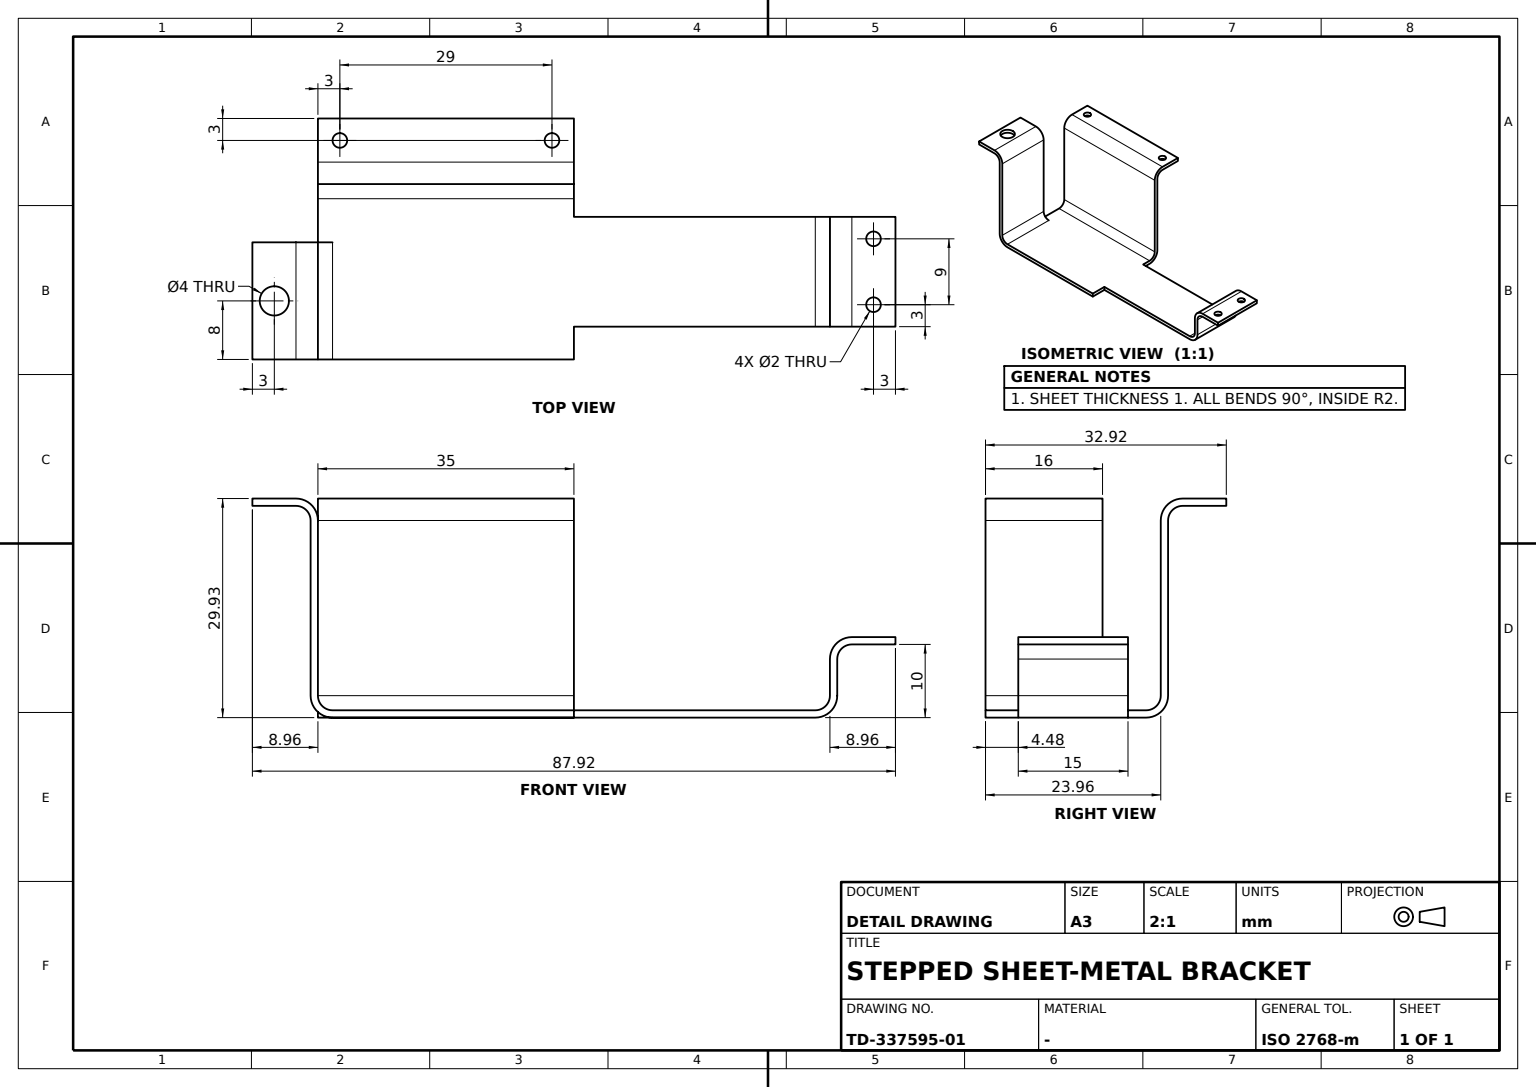
ISO-10303-21;
HEADER;
FILE_DESCRIPTION((''),'2;1');
FILE_NAME('','',(''),(''),'','','');
FILE_SCHEMA(('AUTOMOTIVE_DESIGN'));
ENDSEC;
DATA;
#1=APPLICATION_CONTEXT('');
#2=PRODUCT_CONTEXT('',#1,'mechanical');
#3=PRODUCT('','','',(#2));
#4=PRODUCT_DEFINITION_FORMATION('','',#3);
#5=PRODUCT_DEFINITION_CONTEXT('',#1,'design');
#6=PRODUCT_DEFINITION('','',#4,#5);
#7=PRODUCT_DEFINITION_SHAPE('','',#6);
#8=(LENGTH_UNIT()NAMED_UNIT(*)SI_UNIT(.MILLI.,.METRE.));
#9=(NAMED_UNIT(*)PLANE_ANGLE_UNIT()SI_UNIT($,.RADIAN.));
#10=(NAMED_UNIT(*)SI_UNIT($,.STERADIAN.)SOLID_ANGLE_UNIT());
#11=UNCERTAINTY_MEASURE_WITH_UNIT(LENGTH_MEASURE(0.005),#8,'distance_accuracy_value','');
#12=(GEOMETRIC_REPRESENTATION_CONTEXT(3)GLOBAL_UNCERTAINTY_ASSIGNED_CONTEXT((#11))GLOBAL_UNIT_ASSIGNED_CONTEXT((#8,#9,#10))REPRESENTATION_CONTEXT('',''));
#13=CARTESIAN_POINT('',(18.94,38.,29.93));
#14=VERTEX_POINT('',#13);
#15=CARTESIAN_POINT('',(17.94,38.,29.93));
#16=DIRECTION('',(0.,0.,1.));
#17=DIRECTION('',(1.,0.,0.));
#18=AXIS2_PLACEMENT_3D('',#15,#16,#17);
#19=CIRCLE('',#18,1.);
#20=EDGE_CURVE('',#14,#14,#19,.T.);
#21=ORIENTED_EDGE('',*,*,#20,.T.);
#22=EDGE_LOOP('',(#21));
#23=FACE_BOUND('',#22,.T.);
#24=CARTESIAN_POINT('',(18.94,38.,28.93));
#25=VERTEX_POINT('',#24);
#26=CARTESIAN_POINT('',(17.94,38.,28.93));
#27=AXIS2_PLACEMENT_3D('',#26,#16,#17);
#28=CIRCLE('',#27,1.);
#29=EDGE_CURVE('',#25,#25,#28,.T.);
#30=ORIENTED_EDGE('',*,*,#29,.F.);
#31=EDGE_LOOP('',(#30));
#32=FACE_BOUND('',#31,.T.);
#33=CARTESIAN_POINT('',(17.94,38.,29.43));
#34=DIRECTION('',(0.,0.,-1.));
#35=AXIS2_PLACEMENT_3D('',#33,#34,#17);
#36=CYLINDRICAL_SURFACE('',#35,1.);
#37=ADVANCED_FACE('',(#23,#32),#36,.F.);
#38=CARTESIAN_POINT('',(9.98,35.,0.));
#39=VERTEX_POINT('',#38);
#40=CARTESIAN_POINT('',(9.98,70.,0.));
#41=VERTEX_POINT('',#40);
#42=DIRECTION('',(0.,1.,0.));
#43=VECTOR('',#42,1000.);
#44=LINE('',#38,#43);
#45=EDGE_CURVE('',#39,#41,#44,.T.);
#46=ORIENTED_EDGE('',*,*,#45,.F.);
#47=CARTESIAN_POINT('',(7.5,35.,0.));
#48=VERTEX_POINT('',#47);
#49=CARTESIAN_POINT('',(0.,35.,0.));
#50=VECTOR('',#17,1000.);
#51=LINE('',#49,#50);
#52=EDGE_CURVE('',#48,#39,#51,.T.);
#53=ORIENTED_EDGE('',*,*,#52,.F.);
#54=CARTESIAN_POINT('',(7.5,2.,0.));
#55=VERTEX_POINT('',#54);
#56=CARTESIAN_POINT('',(7.5,0.,0.));
#57=LINE('',#56,#43);
#58=EDGE_CURVE('',#55,#48,#57,.T.);
#59=ORIENTED_EDGE('',*,*,#58,.F.);
#60=CARTESIAN_POINT('',(-7.5,2.,0.));
#61=VERTEX_POINT('',#60);
#62=CARTESIAN_POINT('',(-1.,2.,0.));
#63=LINE('',#62,#50);
#64=EDGE_CURVE('',#61,#55,#63,.T.);
#65=ORIENTED_EDGE('',*,*,#64,.F.);
#66=CARTESIAN_POINT('',(-7.5,35.,0.));
#67=VERTEX_POINT('',#66);
#68=CARTESIAN_POINT('',(-7.5,0.,0.));
#69=LINE('',#68,#43);
#70=EDGE_CURVE('',#67,#61,#69,.F.);
#71=ORIENTED_EDGE('',*,*,#70,.F.);
#72=CARTESIAN_POINT('',(-11.98,35.,0.));
#73=VERTEX_POINT('',#72);
#74=EDGE_CURVE('',#73,#67,#51,.T.);
#75=ORIENTED_EDGE('',*,*,#74,.F.);
#76=CARTESIAN_POINT('',(-11.98,68.,0.));
#77=VERTEX_POINT('',#76);
#78=CARTESIAN_POINT('',(-11.98,0.,0.));
#79=DIRECTION('',(0.,-1.,0.));
#80=VECTOR('',#79,1000.);
#81=LINE('',#78,#80);
#82=EDGE_CURVE('',#77,#73,#81,.T.);
#83=ORIENTED_EDGE('',*,*,#82,.F.);
#84=CARTESIAN_POINT('',(4.02,68.,0.));
#85=VERTEX_POINT('',#84);
#86=CARTESIAN_POINT('',(-1.,68.,0.));
#87=DIRECTION('',(-1.,0.,0.));
#88=VECTOR('',#87,1000.);
#89=LINE('',#86,#88);
#90=EDGE_CURVE('',#85,#77,#89,.T.);
#91=ORIENTED_EDGE('',*,*,#90,.F.);
#92=CARTESIAN_POINT('',(4.02,70.,0.));
#93=VERTEX_POINT('',#92);
#94=CARTESIAN_POINT('',(4.02,0.,0.));
#95=LINE('',#94,#80);
#96=EDGE_CURVE('',#93,#85,#95,.T.);
#97=ORIENTED_EDGE('',*,*,#96,.F.);
#98=CARTESIAN_POINT('',(0.,70.,0.));
#99=LINE('',#98,#88);
#100=EDGE_CURVE('',#41,#93,#99,.T.);
#101=ORIENTED_EDGE('',*,*,#100,.F.);
#102=EDGE_LOOP('',(#46,#53,#59,#65,#71,#75,#83,#91,#97,#101));
#103=FACE_BOUND('',#102,.T.);
#104=CARTESIAN_POINT('',(0.,0.,0.));
#105=AXIS2_PLACEMENT_3D('',#104,#16,#42);
#106=PLANE('',#105);
#107=ADVANCED_FACE('',(#103),#106,.F.);
#108=CARTESIAN_POINT('',(4.02,78.96,28.93));
#109=VERTEX_POINT('',#108);
#110=CARTESIAN_POINT('',(-11.98,78.96,28.93));
#111=VERTEX_POINT('',#110);
#112=CARTESIAN_POINT('',(-3.98,78.96,28.93));
#113=LINE('',#112,#88);
#114=EDGE_CURVE('',#109,#111,#113,.T.);
#115=ORIENTED_EDGE('',*,*,#114,.T.);
#116=CARTESIAN_POINT('',(-11.98,78.96,29.93));
#117=VERTEX_POINT('',#116);
#118=CARTESIAN_POINT('',(-11.98,78.96,0.));
#119=VECTOR('',#16,1000.);
#120=LINE('',#118,#119);
#121=EDGE_CURVE('',#111,#117,#120,.T.);
#122=ORIENTED_EDGE('',*,*,#121,.T.);
#123=CARTESIAN_POINT('',(4.02,78.96,29.93));
#124=VERTEX_POINT('',#123);
#125=CARTESIAN_POINT('',(-3.98,78.96,29.93));
#126=LINE('',#125,#88);
#127=EDGE_CURVE('',#124,#117,#126,.T.);
#128=ORIENTED_EDGE('',*,*,#127,.F.);
#129=CARTESIAN_POINT('',(4.02,78.96,0.));
#130=LINE('',#129,#119);
#131=EDGE_CURVE('',#109,#124,#130,.T.);
#132=ORIENTED_EDGE('',*,*,#131,.F.);
#133=EDGE_LOOP('',(#115,#122,#128,#132));
#134=FACE_BOUND('',#133,.T.);
#135=AXIS2_PLACEMENT_3D('',#125,#79,#17);
#136=PLANE('',#135);
#137=ADVANCED_FACE('',(#134),#136,.F.);
#138=CARTESIAN_POINT('',(-7.5,-3.,10.));
#139=VERTEX_POINT('',#138);
#140=CARTESIAN_POINT('',(7.5,-3.,10.));
#141=VERTEX_POINT('',#140);
#142=CARTESIAN_POINT('',(0.,-3.,10.));
#143=LINE('',#142,#50);
#144=EDGE_CURVE('',#139,#141,#143,.T.);
#145=ORIENTED_EDGE('',*,*,#144,.F.);
#146=CARTESIAN_POINT('',(-7.5,-1.,8.));
#147=VERTEX_POINT('',#146);
#148=CARTESIAN_POINT('',(-7.5,-3.,8.));
#149=AXIS2_PLACEMENT_3D('',#148,#17,#34);
#150=CIRCLE('',#149,2.);
#151=EDGE_CURVE('',#139,#147,#150,.F.);
#152=ORIENTED_EDGE('',*,*,#151,.T.);
#153=CARTESIAN_POINT('',(7.5,-1.,8.));
#154=VERTEX_POINT('',#153);
#155=CARTESIAN_POINT('',(0.,-1.,8.));
#156=LINE('',#155,#50);
#157=EDGE_CURVE('',#147,#154,#156,.T.);
#158=ORIENTED_EDGE('',*,*,#157,.T.);
#159=CARTESIAN_POINT('',(7.5,-3.,8.));
#160=AXIS2_PLACEMENT_3D('',#159,#17,#34);
#161=CIRCLE('',#160,2.);
#162=EDGE_CURVE('',#141,#154,#161,.F.);
#163=ORIENTED_EDGE('',*,*,#162,.F.);
#164=EDGE_LOOP('',(#145,#152,#158,#163));
#165=FACE_BOUND('',#164,.T.);
#166=CARTESIAN_POINT('',(0.,-3.,8.));
#167=AXIS2_PLACEMENT_3D('',#166,#17,#42);
#168=CYLINDRICAL_SURFACE('',#167,2.);
#169=ADVANCED_FACE('',(#165),#168,.F.);
#170=CARTESIAN_POINT('',(20.94,35.,28.93));
#171=VERTEX_POINT('',#170);
#172=CARTESIAN_POINT('',(20.94,35.,29.93));
#173=VERTEX_POINT('',#172);
#174=CARTESIAN_POINT('',(20.94,35.,0.));
#175=VECTOR('',#34,1000.);
#176=LINE('',#174,#175);
#177=EDGE_CURVE('',#171,#173,#176,.F.);
#178=ORIENTED_EDGE('',*,*,#177,.F.);
#179=CARTESIAN_POINT('',(20.94,70.,28.93));
#180=VERTEX_POINT('',#179);
#181=CARTESIAN_POINT('',(20.94,52.5,28.93));
#182=LINE('',#181,#43);
#183=EDGE_CURVE('',#171,#180,#182,.T.);
#184=ORIENTED_EDGE('',*,*,#183,.T.);
#185=CARTESIAN_POINT('',(20.94,70.,29.93));
#186=VERTEX_POINT('',#185);
#187=CARTESIAN_POINT('',(20.94,70.,0.));
#188=LINE('',#187,#119);
#189=EDGE_CURVE('',#180,#186,#188,.T.);
#190=ORIENTED_EDGE('',*,*,#189,.T.);
#191=CARTESIAN_POINT('',(20.94,52.5,29.93));
#192=LINE('',#191,#43);
#193=EDGE_CURVE('',#173,#186,#192,.T.);
#194=ORIENTED_EDGE('',*,*,#193,.F.);
#195=EDGE_LOOP('',(#178,#184,#190,#194));
#196=FACE_BOUND('',#195,.T.);
#197=AXIS2_PLACEMENT_3D('',#191,#87,#42);
#198=PLANE('',#197);
#199=ADVANCED_FACE('',(#196),#198,.F.);
#200=CARTESIAN_POINT('',(14.98,35.,28.93));
#201=VERTEX_POINT('',#200);
#202=CARTESIAN_POINT('',(-11.98,35.,28.93));
#203=LINE('',#202,#88);
#204=EDGE_CURVE('',#201,#171,#203,.F.);
#205=ORIENTED_EDGE('',*,*,#204,.T.);
#206=ORIENTED_EDGE('',*,*,#177,.T.);
#207=CARTESIAN_POINT('',(14.98,35.,29.93));
#208=VERTEX_POINT('',#207);
#209=CARTESIAN_POINT('',(-11.98,35.,29.93));
#210=LINE('',#209,#88);
#211=EDGE_CURVE('',#208,#173,#210,.F.);
#212=ORIENTED_EDGE('',*,*,#211,.F.);
#213=CARTESIAN_POINT('',(11.98,35.,26.93));
#214=VERTEX_POINT('',#213);
#215=CARTESIAN_POINT('',(14.98,35.,26.93));
#216=AXIS2_PLACEMENT_3D('',#215,#79,#34);
#217=CIRCLE('',#216,3.);
#218=EDGE_CURVE('',#208,#214,#217,.T.);
#219=ORIENTED_EDGE('',*,*,#218,.T.);
#220=CARTESIAN_POINT('',(11.98,35.,3.));
#221=VERTEX_POINT('',#220);
#222=CARTESIAN_POINT('',(11.98,35.,0.));
#223=LINE('',#222,#119);
#224=EDGE_CURVE('',#221,#214,#223,.T.);
#225=ORIENTED_EDGE('',*,*,#224,.F.);
#226=CARTESIAN_POINT('',(9.98,35.,1.));
#227=VERTEX_POINT('',#226);
#228=CARTESIAN_POINT('',(9.98,35.,3.));
#229=AXIS2_PLACEMENT_3D('',#228,#79,#34);
#230=CIRCLE('',#229,2.);
#231=EDGE_CURVE('',#221,#227,#230,.F.);
#232=ORIENTED_EDGE('',*,*,#231,.T.);
#233=CARTESIAN_POINT('',(7.5,35.,1.));
#234=VERTEX_POINT('',#233);
#235=CARTESIAN_POINT('',(0.,35.,1.));
#236=LINE('',#235,#50);
#237=EDGE_CURVE('',#234,#227,#236,.T.);
#238=ORIENTED_EDGE('',*,*,#237,.F.);
#239=CARTESIAN_POINT('',(7.5,35.,11.));
#240=LINE('',#239,#175);
#241=EDGE_CURVE('',#234,#48,#240,.T.);
#242=ORIENTED_EDGE('',*,*,#241,.T.);
#243=ORIENTED_EDGE('',*,*,#52,.T.);
#244=CARTESIAN_POINT('',(12.98,35.,3.));
#245=VERTEX_POINT('',#244);
#246=CIRCLE('',#229,3.);
#247=EDGE_CURVE('',#245,#39,#246,.F.);
#248=ORIENTED_EDGE('',*,*,#247,.F.);
#249=CARTESIAN_POINT('',(12.98,35.,26.93));
#250=VERTEX_POINT('',#249);
#251=CARTESIAN_POINT('',(12.98,35.,1.));
#252=LINE('',#251,#175);
#253=EDGE_CURVE('',#250,#245,#252,.T.);
#254=ORIENTED_EDGE('',*,*,#253,.F.);
#255=CIRCLE('',#216,2.);
#256=EDGE_CURVE('',#201,#250,#255,.T.);
#257=ORIENTED_EDGE('',*,*,#256,.F.);
#258=EDGE_LOOP('',(#205,#206,#212,#219,#225,#232,#238,#242,#243,#248,#254,#257));
#259=FACE_BOUND('',#258,.T.);
#260=AXIS2_PLACEMENT_3D('',#72,#79,#17);
#261=PLANE('',#260);
#262=ADVANCED_FACE('',(#259),#261,.T.);
#263=CARTESIAN_POINT('',(-7.5,0.,3.));
#264=VERTEX_POINT('',#263);
#265=CARTESIAN_POINT('',(-7.5,2.,1.));
#266=VERTEX_POINT('',#265);
#267=CARTESIAN_POINT('',(-7.5,2.,3.));
#268=AXIS2_PLACEMENT_3D('',#267,#17,#34);
#269=CIRCLE('',#268,2.);
#270=EDGE_CURVE('',#264,#266,#269,.T.);
#271=ORIENTED_EDGE('',*,*,#270,.F.);
#272=CARTESIAN_POINT('',(7.5,0.,3.));
#273=VERTEX_POINT('',#272);
#274=CARTESIAN_POINT('',(-1.,0.,3.));
#275=LINE('',#274,#50);
#276=EDGE_CURVE('',#264,#273,#275,.T.);
#277=ORIENTED_EDGE('',*,*,#276,.T.);
#278=CARTESIAN_POINT('',(7.5,2.,1.));
#279=VERTEX_POINT('',#278);
#280=CARTESIAN_POINT('',(7.5,2.,3.));
#281=AXIS2_PLACEMENT_3D('',#280,#17,#34);
#282=CIRCLE('',#281,2.);
#283=EDGE_CURVE('',#273,#279,#282,.T.);
#284=ORIENTED_EDGE('',*,*,#283,.T.);
#285=CARTESIAN_POINT('',(-1.,2.,1.));
#286=LINE('',#285,#50);
#287=EDGE_CURVE('',#266,#279,#286,.T.);
#288=ORIENTED_EDGE('',*,*,#287,.F.);
#289=EDGE_LOOP('',(#271,#277,#284,#288));
#290=FACE_BOUND('',#289,.T.);
#291=CARTESIAN_POINT('',(-1.,2.,3.));
#292=AXIS2_PLACEMENT_3D('',#291,#17,#34);
#293=CYLINDRICAL_SURFACE('',#292,2.);
#294=ADVANCED_FACE('',(#290),#293,.F.);
#295=CARTESIAN_POINT('',(14.98,70.,29.93));
#296=VERTEX_POINT('',#295);
#297=CARTESIAN_POINT('',(14.98,52.5,29.93));
#298=LINE('',#297,#80);
#299=EDGE_CURVE('',#296,#208,#298,.T.);
#300=ORIENTED_EDGE('',*,*,#299,.T.);
#301=ORIENTED_EDGE('',*,*,#211,.T.);
#302=ORIENTED_EDGE('',*,*,#193,.T.);
#303=CARTESIAN_POINT('',(12.98,70.,29.93));
#304=LINE('',#303,#88);
#305=EDGE_CURVE('',#186,#296,#304,.T.);
#306=ORIENTED_EDGE('',*,*,#305,.T.);
#307=EDGE_LOOP('',(#300,#301,#302,#306));
#308=FACE_BOUND('',#307,.T.);
#309=ORIENTED_EDGE('',*,*,#20,.F.);
#310=EDGE_LOOP('',(#309));
#311=FACE_BOUND('',#310,.T.);
#312=CARTESIAN_POINT('',(18.94,67.,29.93));
#313=VERTEX_POINT('',#312);
#314=CARTESIAN_POINT('',(17.94,67.,29.93));
#315=AXIS2_PLACEMENT_3D('',#314,#16,#17);
#316=CIRCLE('',#315,1.);
#317=EDGE_CURVE('',#313,#313,#316,.T.);
#318=ORIENTED_EDGE('',*,*,#317,.F.);
#319=EDGE_LOOP('',(#318));
#320=FACE_BOUND('',#319,.T.);
#321=CARTESIAN_POINT('',(12.98,52.5,29.93));
#322=AXIS2_PLACEMENT_3D('',#321,#16,#79);
#323=PLANE('',#322);
#324=ADVANCED_FACE('',(#308,#311,#320),#323,.T.);
#325=CARTESIAN_POINT('',(4.02,70.,3.));
#326=VERTEX_POINT('',#325);
#327=CARTESIAN_POINT('',(4.02,70.,26.93));
#328=VERTEX_POINT('',#327);
#329=LINE('',#92,#175);
#330=EDGE_CURVE('',#326,#328,#329,.F.);
#331=ORIENTED_EDGE('',*,*,#330,.F.);
#332=CARTESIAN_POINT('',(4.02,68.,1.));
#333=VERTEX_POINT('',#332);
#334=CARTESIAN_POINT('',(4.02,68.,3.));
#335=AXIS2_PLACEMENT_3D('',#334,#87,#16);
#336=CIRCLE('',#335,2.);
#337=EDGE_CURVE('',#333,#326,#336,.F.);
#338=ORIENTED_EDGE('',*,*,#337,.F.);
#339=LINE('',#84,#175);
#340=EDGE_CURVE('',#85,#333,#339,.F.);
#341=ORIENTED_EDGE('',*,*,#340,.F.);
#342=CARTESIAN_POINT('',(4.02,71.,3.));
#343=VERTEX_POINT('',#342);
#344=CIRCLE('',#335,3.);
#345=EDGE_CURVE('',#85,#343,#344,.F.);
#346=ORIENTED_EDGE('',*,*,#345,.T.);
#347=CARTESIAN_POINT('',(4.02,71.,26.93));
#348=VERTEX_POINT('',#347);
#349=CARTESIAN_POINT('',(4.02,71.,1.));
#350=LINE('',#349,#119);
#351=EDGE_CURVE('',#348,#343,#350,.F.);
#352=ORIENTED_EDGE('',*,*,#351,.F.);
#353=CARTESIAN_POINT('',(4.02,73.,28.93));
#354=VERTEX_POINT('',#353);
#355=CARTESIAN_POINT('',(4.02,73.,26.93));
#356=AXIS2_PLACEMENT_3D('',#355,#87,#16);
#357=CIRCLE('',#356,2.);
#358=EDGE_CURVE('',#354,#348,#357,.F.);
#359=ORIENTED_EDGE('',*,*,#358,.F.);
#360=CARTESIAN_POINT('',(4.02,69.,28.93));
#361=LINE('',#360,#43);
#362=EDGE_CURVE('',#354,#109,#361,.T.);
#363=ORIENTED_EDGE('',*,*,#362,.T.);
#364=ORIENTED_EDGE('',*,*,#131,.T.);
#365=CARTESIAN_POINT('',(4.02,73.,29.93));
#366=VERTEX_POINT('',#365);
#367=CARTESIAN_POINT('',(4.02,69.,29.93));
#368=LINE('',#367,#43);
#369=EDGE_CURVE('',#366,#124,#368,.T.);
#370=ORIENTED_EDGE('',*,*,#369,.F.);
#371=CIRCLE('',#356,3.);
#372=EDGE_CURVE('',#366,#328,#371,.F.);
#373=ORIENTED_EDGE('',*,*,#372,.T.);
#374=EDGE_LOOP('',(#331,#338,#341,#346,#352,#359,#363,#364,#370,#373));
#375=FACE_BOUND('',#374,.T.);
#376=CARTESIAN_POINT('',(4.02,69.,0.));
#377=AXIS2_PLACEMENT_3D('',#376,#87,#42);
#378=PLANE('',#377);
#379=ADVANCED_FACE('',(#375),#378,.F.);
#380=CARTESIAN_POINT('',(-11.98,73.,29.93));
#381=VERTEX_POINT('',#380);
#382=CARTESIAN_POINT('',(-11.98,70.,26.93));
#383=VERTEX_POINT('',#382);
#384=CARTESIAN_POINT('',(-11.98,73.,26.93));
#385=AXIS2_PLACEMENT_3D('',#384,#87,#16);
#386=CIRCLE('',#385,3.);
#387=EDGE_CURVE('',#381,#383,#386,.F.);
#388=ORIENTED_EDGE('',*,*,#387,.T.);
#389=CARTESIAN_POINT('',(-3.98,70.,26.93));
#390=LINE('',#389,#88);
#391=EDGE_CURVE('',#328,#383,#390,.T.);
#392=ORIENTED_EDGE('',*,*,#391,.F.);
#393=ORIENTED_EDGE('',*,*,#372,.F.);
#394=CARTESIAN_POINT('',(-3.98,73.,29.93));
#395=LINE('',#394,#88);
#396=EDGE_CURVE('',#366,#381,#395,.T.);
#397=ORIENTED_EDGE('',*,*,#396,.T.);
#398=EDGE_LOOP('',(#388,#392,#393,#397));
#399=FACE_BOUND('',#398,.T.);
#400=CARTESIAN_POINT('',(-3.98,73.,26.93));
#401=AXIS2_PLACEMENT_3D('',#400,#87,#79);
#402=CYLINDRICAL_SURFACE('',#401,3.);
#403=ADVANCED_FACE('',(#399),#402,.T.);
#404=CARTESIAN_POINT('',(18.94,67.,28.93));
#405=VERTEX_POINT('',#404);
#406=CARTESIAN_POINT('',(17.94,67.,28.93));
#407=AXIS2_PLACEMENT_3D('',#406,#16,#17);
#408=CIRCLE('',#407,1.);
#409=EDGE_CURVE('',#405,#405,#408,.T.);
#410=ORIENTED_EDGE('',*,*,#409,.T.);
#411=EDGE_LOOP('',(#410));
#412=FACE_BOUND('',#411,.T.);
#413=CARTESIAN_POINT('',(14.98,70.,28.93));
#414=VERTEX_POINT('',#413);
#415=CARTESIAN_POINT('',(12.98,70.,28.93));
#416=LINE('',#415,#88);
#417=EDGE_CURVE('',#180,#414,#416,.T.);
#418=ORIENTED_EDGE('',*,*,#417,.F.);
#419=ORIENTED_EDGE('',*,*,#183,.F.);
#420=ORIENTED_EDGE('',*,*,#204,.F.);
#421=CARTESIAN_POINT('',(14.98,52.5,28.93));
#422=LINE('',#421,#80);
#423=EDGE_CURVE('',#414,#201,#422,.T.);
#424=ORIENTED_EDGE('',*,*,#423,.F.);
#425=EDGE_LOOP('',(#418,#419,#420,#424));
#426=FACE_BOUND('',#425,.T.);
#427=ORIENTED_EDGE('',*,*,#29,.T.);
#428=EDGE_LOOP('',(#427));
#429=FACE_BOUND('',#428,.T.);
#430=CARTESIAN_POINT('',(12.98,52.5,28.93));
#431=AXIS2_PLACEMENT_3D('',#430,#16,#79);
#432=PLANE('',#431);
#433=ADVANCED_FACE('',(#412,#426,#429),#432,.F.);
#434=ORIENTED_EDGE('',*,*,#330,.T.);
#435=ORIENTED_EDGE('',*,*,#391,.T.);
#436=CARTESIAN_POINT('',(-11.98,70.,3.));
#437=VERTEX_POINT('',#436);
#438=CARTESIAN_POINT('',(-11.98,70.,0.));
#439=LINE('',#438,#175);
#440=EDGE_CURVE('',#437,#383,#439,.F.);
#441=ORIENTED_EDGE('',*,*,#440,.F.);
#442=CARTESIAN_POINT('',(-1.,70.,3.));
#443=LINE('',#442,#88);
#444=EDGE_CURVE('',#326,#437,#443,.T.);
#445=ORIENTED_EDGE('',*,*,#444,.F.);
#446=EDGE_LOOP('',(#434,#435,#441,#445));
#447=FACE_BOUND('',#446,.T.);
#448=CARTESIAN_POINT('',(11.98,70.,0.));
#449=AXIS2_PLACEMENT_3D('',#448,#42,#87);
#450=PLANE('',#449);
#451=ADVANCED_FACE('',(#447),#450,.F.);
#452=CARTESIAN_POINT('',(12.98,70.,26.93));
#453=VERTEX_POINT('',#452);
#454=CARTESIAN_POINT('',(14.98,70.,26.93));
#455=AXIS2_PLACEMENT_3D('',#454,#42,#16);
#456=CIRCLE('',#455,2.);
#457=EDGE_CURVE('',#414,#453,#456,.F.);
#458=ORIENTED_EDGE('',*,*,#457,.T.);
#459=CARTESIAN_POINT('',(12.98,70.,3.));
#460=VERTEX_POINT('',#459);
#461=CARTESIAN_POINT('',(12.98,70.,1.));
#462=LINE('',#461,#119);
#463=EDGE_CURVE('',#453,#460,#462,.F.);
#464=ORIENTED_EDGE('',*,*,#463,.T.);
#465=CARTESIAN_POINT('',(9.98,70.,3.));
#466=AXIS2_PLACEMENT_3D('',#465,#42,#16);
#467=CIRCLE('',#466,3.);
#468=EDGE_CURVE('',#460,#41,#467,.T.);
#469=ORIENTED_EDGE('',*,*,#468,.T.);
#470=ORIENTED_EDGE('',*,*,#100,.T.);
#471=CARTESIAN_POINT('',(4.02,70.,1.));
#472=VERTEX_POINT('',#471);
#473=LINE('',#92,#119);
#474=EDGE_CURVE('',#93,#472,#473,.T.);
#475=ORIENTED_EDGE('',*,*,#474,.T.);
#476=CARTESIAN_POINT('',(9.98,70.,1.));
#477=VERTEX_POINT('',#476);
#478=CARTESIAN_POINT('',(0.,70.,1.));
#479=LINE('',#478,#88);
#480=EDGE_CURVE('',#477,#472,#479,.T.);
#481=ORIENTED_EDGE('',*,*,#480,.F.);
#482=CARTESIAN_POINT('',(11.98,70.,3.));
#483=VERTEX_POINT('',#482);
#484=CIRCLE('',#466,2.);
#485=EDGE_CURVE('',#483,#477,#484,.T.);
#486=ORIENTED_EDGE('',*,*,#485,.F.);
#487=CARTESIAN_POINT('',(11.98,70.,26.93));
#488=VERTEX_POINT('',#487);
#489=LINE('',#448,#175);
#490=EDGE_CURVE('',#483,#488,#489,.F.);
#491=ORIENTED_EDGE('',*,*,#490,.T.);
#492=CIRCLE('',#455,3.);
#493=EDGE_CURVE('',#296,#488,#492,.F.);
#494=ORIENTED_EDGE('',*,*,#493,.F.);
#495=ORIENTED_EDGE('',*,*,#305,.F.);
#496=ORIENTED_EDGE('',*,*,#189,.F.);
#497=ORIENTED_EDGE('',*,*,#417,.T.);
#498=EDGE_LOOP('',(#458,#464,#469,#470,#475,#481,#486,#491,#494,#495,#496,#497));
#499=FACE_BOUND('',#498,.T.);
#500=ADVANCED_FACE('',(#499),#450,.T.);
#501=LINE('',#220,#43);
#502=EDGE_CURVE('',#221,#483,#501,.T.);
#503=ORIENTED_EDGE('',*,*,#502,.T.);
#504=ORIENTED_EDGE('',*,*,#485,.T.);
#505=LINE('',#226,#43);
#506=EDGE_CURVE('',#227,#477,#505,.T.);
#507=ORIENTED_EDGE('',*,*,#506,.F.);
#508=ORIENTED_EDGE('',*,*,#231,.F.);
#509=EDGE_LOOP('',(#503,#504,#507,#508));
#510=FACE_BOUND('',#509,.T.);
#511=AXIS2_PLACEMENT_3D('',#228,#42,#34);
#512=CYLINDRICAL_SURFACE('',#511,2.);
#513=ADVANCED_FACE('',(#510),#512,.F.);
#514=ORIENTED_EDGE('',*,*,#58,.T.);
#515=ORIENTED_EDGE('',*,*,#241,.F.);
#516=CARTESIAN_POINT('',(7.5,0.,1.));
#517=LINE('',#516,#43);
#518=EDGE_CURVE('',#279,#234,#517,.T.);
#519=ORIENTED_EDGE('',*,*,#518,.F.);
#520=ORIENTED_EDGE('',*,*,#283,.F.);
#521=CARTESIAN_POINT('',(7.5,0.,8.));
#522=VERTEX_POINT('',#521);
#523=CARTESIAN_POINT('',(7.5,0.,11.));
#524=LINE('',#523,#175);
#525=EDGE_CURVE('',#273,#522,#524,.F.);
#526=ORIENTED_EDGE('',*,*,#525,.T.);
#527=CARTESIAN_POINT('',(7.5,-3.,11.));
#528=VERTEX_POINT('',#527);
#529=CIRCLE('',#160,3.);
#530=EDGE_CURVE('',#528,#522,#529,.F.);
#531=ORIENTED_EDGE('',*,*,#530,.F.);
#532=CARTESIAN_POINT('',(7.5,-8.96,11.));
#533=VERTEX_POINT('',#532);
#534=CARTESIAN_POINT('',(7.5,-1.,11.));
#535=LINE('',#534,#43);
#536=EDGE_CURVE('',#533,#528,#535,.T.);
#537=ORIENTED_EDGE('',*,*,#536,.F.);
#538=CARTESIAN_POINT('',(7.5,-8.96,10.));
#539=VERTEX_POINT('',#538);
#540=LINE('',#532,#119);
#541=EDGE_CURVE('',#539,#533,#540,.T.);
#542=ORIENTED_EDGE('',*,*,#541,.F.);
#543=CARTESIAN_POINT('',(7.5,-1.,10.));
#544=LINE('',#543,#43);
#545=EDGE_CURVE('',#539,#141,#544,.T.);
#546=ORIENTED_EDGE('',*,*,#545,.T.);
#547=ORIENTED_EDGE('',*,*,#162,.T.);
#548=CARTESIAN_POINT('',(7.5,-1.,3.));
#549=VERTEX_POINT('',#548);
#550=CARTESIAN_POINT('',(7.5,-1.,1.));
#551=LINE('',#550,#119);
#552=EDGE_CURVE('',#154,#549,#551,.F.);
#553=ORIENTED_EDGE('',*,*,#552,.T.);
#554=CIRCLE('',#281,3.);
#555=EDGE_CURVE('',#549,#55,#554,.T.);
#556=ORIENTED_EDGE('',*,*,#555,.T.);
#557=EDGE_LOOP('',(#514,#515,#519,#520,#526,#531,#537,#542,#546,#547,#553,#556));
#558=FACE_BOUND('',#557,.T.);
#559=CARTESIAN_POINT('',(7.5,-5.98,11.));
#560=AXIS2_PLACEMENT_3D('',#559,#17,#42);
#561=PLANE('',#560);
#562=ADVANCED_FACE('',(#558),#561,.T.);
#563=CARTESIAN_POINT('',(-7.5,-1.,3.));
#564=VERTEX_POINT('',#563);
#565=CARTESIAN_POINT('',(-7.5,-1.,1.));
#566=LINE('',#565,#119);
#567=EDGE_CURVE('',#147,#564,#566,.F.);
#568=ORIENTED_EDGE('',*,*,#567,.T.);
#569=CARTESIAN_POINT('',(-1.,-1.,3.));
#570=LINE('',#569,#50);
#571=EDGE_CURVE('',#564,#549,#570,.T.);
#572=ORIENTED_EDGE('',*,*,#571,.T.);
#573=ORIENTED_EDGE('',*,*,#552,.F.);
#574=ORIENTED_EDGE('',*,*,#157,.F.);
#575=EDGE_LOOP('',(#568,#572,#573,#574));
#576=FACE_BOUND('',#575,.T.);
#577=CARTESIAN_POINT('',(0.,-1.,1.));
#578=AXIS2_PLACEMENT_3D('',#577,#79,#17);
#579=PLANE('',#578);
#580=ADVANCED_FACE('',(#576),#579,.T.);
#581=CARTESIAN_POINT('',(11.98,52.5,26.93));
#582=LINE('',#581,#80);
#583=EDGE_CURVE('',#488,#214,#582,.T.);
#584=ORIENTED_EDGE('',*,*,#583,.F.);
#585=ORIENTED_EDGE('',*,*,#490,.F.);
#586=ORIENTED_EDGE('',*,*,#502,.F.);
#587=ORIENTED_EDGE('',*,*,#224,.T.);
#588=EDGE_LOOP('',(#584,#585,#586,#587));
#589=FACE_BOUND('',#588,.T.);
#590=CARTESIAN_POINT('',(11.98,52.5,1.));
#591=AXIS2_PLACEMENT_3D('',#590,#17,#42);
#592=PLANE('',#591);
#593=ADVANCED_FACE('',(#589),#592,.F.);
#594=ORIENTED_EDGE('',*,*,#423,.T.);
#595=ORIENTED_EDGE('',*,*,#256,.T.);
#596=CARTESIAN_POINT('',(12.98,52.5,26.93));
#597=LINE('',#596,#80);
#598=EDGE_CURVE('',#453,#250,#597,.T.);
#599=ORIENTED_EDGE('',*,*,#598,.F.);
#600=ORIENTED_EDGE('',*,*,#457,.F.);
#601=EDGE_LOOP('',(#594,#595,#599,#600));
#602=FACE_BOUND('',#601,.T.);
#603=CARTESIAN_POINT('',(14.98,52.5,26.93));
#604=AXIS2_PLACEMENT_3D('',#603,#79,#87);
#605=CYLINDRICAL_SURFACE('',#604,2.);
#606=ADVANCED_FACE('',(#602),#605,.F.);
#607=ORIENTED_EDGE('',*,*,#317,.T.);
#608=EDGE_LOOP('',(#607));
#609=FACE_BOUND('',#608,.T.);
#610=ORIENTED_EDGE('',*,*,#409,.F.);
#611=EDGE_LOOP('',(#610));
#612=FACE_BOUND('',#611,.T.);
#613=CARTESIAN_POINT('',(17.94,67.,29.43));
#614=AXIS2_PLACEMENT_3D('',#613,#34,#17);
#615=CYLINDRICAL_SURFACE('',#614,1.);
#616=ADVANCED_FACE('',(#609,#612),#615,.F.);
#617=ORIENTED_EDGE('',*,*,#583,.T.);
#618=ORIENTED_EDGE('',*,*,#218,.F.);
#619=ORIENTED_EDGE('',*,*,#299,.F.);
#620=ORIENTED_EDGE('',*,*,#493,.T.);
#621=EDGE_LOOP('',(#617,#618,#619,#620));
#622=FACE_BOUND('',#621,.T.);
#623=CYLINDRICAL_SURFACE('',#604,3.);
#624=ADVANCED_FACE('',(#622),#623,.T.);
#625=CARTESIAN_POINT('',(-1.98,75.96,28.93));
#626=VERTEX_POINT('',#625);
#627=CARTESIAN_POINT('',(-3.98,75.96,28.93));
#628=AXIS2_PLACEMENT_3D('',#627,#16,#17);
#629=CIRCLE('',#628,2.);
#630=EDGE_CURVE('',#626,#626,#629,.T.);
#631=ORIENTED_EDGE('',*,*,#630,.T.);
#632=EDGE_LOOP('',(#631));
#633=FACE_BOUND('',#632,.T.);
#634=CARTESIAN_POINT('',(-11.98,73.,28.93));
#635=VERTEX_POINT('',#634);
#636=CARTESIAN_POINT('',(-3.98,73.,28.93));
#637=LINE('',#636,#88);
#638=EDGE_CURVE('',#354,#635,#637,.T.);
#639=ORIENTED_EDGE('',*,*,#638,.T.);
#640=CARTESIAN_POINT('',(-11.98,52.5,28.93));
#641=LINE('',#640,#80);
#642=EDGE_CURVE('',#111,#635,#641,.T.);
#643=ORIENTED_EDGE('',*,*,#642,.F.);
#644=ORIENTED_EDGE('',*,*,#114,.F.);
#645=ORIENTED_EDGE('',*,*,#362,.F.);
#646=EDGE_LOOP('',(#639,#643,#644,#645));
#647=FACE_BOUND('',#646,.T.);
#648=ADVANCED_FACE('',(#633,#647),#432,.F.);
#649=CARTESIAN_POINT('',(-11.98,68.,1.));
#650=VERTEX_POINT('',#649);
#651=CARTESIAN_POINT('',(-11.98,68.,3.));
#652=AXIS2_PLACEMENT_3D('',#651,#87,#16);
#653=CIRCLE('',#652,2.);
#654=EDGE_CURVE('',#437,#650,#653,.T.);
#655=ORIENTED_EDGE('',*,*,#654,.T.);
#656=CARTESIAN_POINT('',(-1.,68.,1.));
#657=LINE('',#656,#88);
#658=EDGE_CURVE('',#333,#650,#657,.T.);
#659=ORIENTED_EDGE('',*,*,#658,.F.);
#660=ORIENTED_EDGE('',*,*,#337,.T.);
#661=ORIENTED_EDGE('',*,*,#444,.T.);
#662=EDGE_LOOP('',(#655,#659,#660,#661));
#663=FACE_BOUND('',#662,.T.);
#664=CARTESIAN_POINT('',(-1.,68.,3.));
#665=AXIS2_PLACEMENT_3D('',#664,#87,#34);
#666=CYLINDRICAL_SURFACE('',#665,2.);
#667=ADVANCED_FACE('',(#663),#666,.F.);
#668=ORIENTED_EDGE('',*,*,#598,.T.);
#669=ORIENTED_EDGE('',*,*,#253,.T.);
#670=LINE('',#244,#43);
#671=EDGE_CURVE('',#245,#460,#670,.T.);
#672=ORIENTED_EDGE('',*,*,#671,.T.);
#673=ORIENTED_EDGE('',*,*,#463,.F.);
#674=EDGE_LOOP('',(#668,#669,#672,#673));
#675=FACE_BOUND('',#674,.T.);
#676=CARTESIAN_POINT('',(12.98,52.5,1.));
#677=AXIS2_PLACEMENT_3D('',#676,#17,#42);
#678=PLANE('',#677);
#679=ADVANCED_FACE('',(#675),#678,.T.);
#680=CARTESIAN_POINT('',(4.02,0.,1.));
#681=LINE('',#680,#80);
#682=EDGE_CURVE('',#472,#333,#681,.T.);
#683=ORIENTED_EDGE('',*,*,#682,.T.);
#684=ORIENTED_EDGE('',*,*,#658,.T.);
#685=CARTESIAN_POINT('',(-11.98,35.,1.));
#686=VERTEX_POINT('',#685);
#687=CARTESIAN_POINT('',(-11.98,0.,1.));
#688=LINE('',#687,#80);
#689=EDGE_CURVE('',#650,#686,#688,.T.);
#690=ORIENTED_EDGE('',*,*,#689,.T.);
#691=CARTESIAN_POINT('',(-7.5,35.,1.));
#692=VERTEX_POINT('',#691);
#693=EDGE_CURVE('',#686,#692,#236,.T.);
#694=ORIENTED_EDGE('',*,*,#693,.T.);
#695=CARTESIAN_POINT('',(-7.5,0.,1.));
#696=LINE('',#695,#43);
#697=EDGE_CURVE('',#692,#266,#696,.F.);
#698=ORIENTED_EDGE('',*,*,#697,.T.);
#699=ORIENTED_EDGE('',*,*,#287,.T.);
#700=ORIENTED_EDGE('',*,*,#518,.T.);
#701=ORIENTED_EDGE('',*,*,#237,.T.);
#702=ORIENTED_EDGE('',*,*,#506,.T.);
#703=ORIENTED_EDGE('',*,*,#480,.T.);
#704=EDGE_LOOP('',(#683,#684,#690,#694,#698,#699,#700,#701,#702,#703));
#705=FACE_BOUND('',#704,.T.);
#706=CARTESIAN_POINT('',(0.,0.,1.));
#707=AXIS2_PLACEMENT_3D('',#706,#16,#42);
#708=PLANE('',#707);
#709=ADVANCED_FACE('',(#705),#708,.T.);
#710=ORIENTED_EDGE('',*,*,#247,.T.);
#711=ORIENTED_EDGE('',*,*,#45,.T.);
#712=ORIENTED_EDGE('',*,*,#468,.F.);
#713=ORIENTED_EDGE('',*,*,#671,.F.);
#714=EDGE_LOOP('',(#710,#711,#712,#713));
#715=FACE_BOUND('',#714,.T.);
#716=CYLINDRICAL_SURFACE('',#511,3.);
#717=ADVANCED_FACE('',(#715),#716,.T.);
#718=CARTESIAN_POINT('',(-1.98,75.96,29.93));
#719=VERTEX_POINT('',#718);
#720=CARTESIAN_POINT('',(-3.98,75.96,29.93));
#721=AXIS2_PLACEMENT_3D('',#720,#16,#17);
#722=CIRCLE('',#721,2.);
#723=EDGE_CURVE('',#719,#719,#722,.T.);
#724=ORIENTED_EDGE('',*,*,#723,.T.);
#725=EDGE_LOOP('',(#724));
#726=FACE_BOUND('',#725,.T.);
#727=ORIENTED_EDGE('',*,*,#630,.F.);
#728=EDGE_LOOP('',(#727));
#729=FACE_BOUND('',#728,.T.);
#730=CARTESIAN_POINT('',(-3.98,75.96,29.43));
#731=AXIS2_PLACEMENT_3D('',#730,#34,#17);
#732=CYLINDRICAL_SURFACE('',#731,2.);
#733=ADVANCED_FACE('',(#726,#729),#732,.F.);
#734=CARTESIAN_POINT('',(5.5,-5.96,10.));
#735=VERTEX_POINT('',#734);
#736=CARTESIAN_POINT('',(4.5,-5.96,10.));
#737=AXIS2_PLACEMENT_3D('',#736,#16,#17);
#738=CIRCLE('',#737,1.);
#739=EDGE_CURVE('',#735,#735,#738,.T.);
#740=ORIENTED_EDGE('',*,*,#739,.T.);
#741=EDGE_LOOP('',(#740));
#742=FACE_BOUND('',#741,.T.);
#743=ORIENTED_EDGE('',*,*,#144,.T.);
#744=ORIENTED_EDGE('',*,*,#545,.F.);
#745=CARTESIAN_POINT('',(-7.5,-8.96,10.));
#746=VERTEX_POINT('',#745);
#747=CARTESIAN_POINT('',(0.,-8.96,10.));
#748=LINE('',#747,#50);
#749=EDGE_CURVE('',#746,#539,#748,.T.);
#750=ORIENTED_EDGE('',*,*,#749,.F.);
#751=CARTESIAN_POINT('',(-7.5,-5.98,10.));
#752=LINE('',#751,#80);
#753=EDGE_CURVE('',#139,#746,#752,.T.);
#754=ORIENTED_EDGE('',*,*,#753,.F.);
#755=EDGE_LOOP('',(#743,#744,#750,#754));
#756=FACE_BOUND('',#755,.T.);
#757=CARTESIAN_POINT('',(-3.5,-5.96,10.));
#758=VERTEX_POINT('',#757);
#759=CARTESIAN_POINT('',(-4.5,-5.96,10.));
#760=AXIS2_PLACEMENT_3D('',#759,#16,#17);
#761=CIRCLE('',#760,1.);
#762=EDGE_CURVE('',#758,#758,#761,.T.);
#763=ORIENTED_EDGE('',*,*,#762,.T.);
#764=EDGE_LOOP('',(#763));
#765=FACE_BOUND('',#764,.T.);
#766=CARTESIAN_POINT('',(0.,-1.,10.));
#767=AXIS2_PLACEMENT_3D('',#766,#16,#87);
#768=PLANE('',#767);
#769=ADVANCED_FACE('',(#742,#756,#765),#768,.F.);
#770=LINE('',#66,#119);
#771=EDGE_CURVE('',#692,#67,#770,.F.);
#772=ORIENTED_EDGE('',*,*,#771,.F.);
#773=ORIENTED_EDGE('',*,*,#693,.F.);
#774=LINE('',#72,#175);
#775=EDGE_CURVE('',#686,#73,#774,.T.);
#776=ORIENTED_EDGE('',*,*,#775,.T.);
#777=ORIENTED_EDGE('',*,*,#74,.T.);
#778=EDGE_LOOP('',(#772,#773,#776,#777));
#779=FACE_BOUND('',#778,.T.);
#780=ADVANCED_FACE('',(#779),#261,.T.);
#781=CARTESIAN_POINT('',(-11.98,71.,26.93));
#782=VERTEX_POINT('',#781);
#783=CIRCLE('',#385,2.);
#784=EDGE_CURVE('',#635,#782,#783,.F.);
#785=ORIENTED_EDGE('',*,*,#784,.T.);
#786=CARTESIAN_POINT('',(-11.98,71.,3.));
#787=VERTEX_POINT('',#786);
#788=CARTESIAN_POINT('',(-11.98,71.,1.));
#789=LINE('',#788,#119);
#790=EDGE_CURVE('',#782,#787,#789,.F.);
#791=ORIENTED_EDGE('',*,*,#790,.T.);
#792=CIRCLE('',#652,3.);
#793=EDGE_CURVE('',#787,#77,#792,.T.);
#794=ORIENTED_EDGE('',*,*,#793,.T.);
#795=ORIENTED_EDGE('',*,*,#82,.T.);
#796=ORIENTED_EDGE('',*,*,#775,.F.);
#797=ORIENTED_EDGE('',*,*,#689,.F.);
#798=ORIENTED_EDGE('',*,*,#654,.F.);
#799=ORIENTED_EDGE('',*,*,#440,.T.);
#800=ORIENTED_EDGE('',*,*,#387,.F.);
#801=CARTESIAN_POINT('',(-11.98,52.5,29.93));
#802=LINE('',#801,#80);
#803=EDGE_CURVE('',#117,#381,#802,.T.);
#804=ORIENTED_EDGE('',*,*,#803,.F.);
#805=ORIENTED_EDGE('',*,*,#121,.F.);
#806=ORIENTED_EDGE('',*,*,#642,.T.);
#807=EDGE_LOOP('',(#785,#791,#794,#795,#796,#797,#798,#799,#800,#804,#805,#806));
#808=FACE_BOUND('',#807,.T.);
#809=AXIS2_PLACEMENT_3D('',#438,#87,#79);
#810=PLANE('',#809);
#811=ADVANCED_FACE('',(#808),#810,.T.);
#812=CIRCLE('',#268,3.);
#813=EDGE_CURVE('',#564,#61,#812,.T.);
#814=ORIENTED_EDGE('',*,*,#813,.T.);
#815=ORIENTED_EDGE('',*,*,#64,.T.);
#816=ORIENTED_EDGE('',*,*,#555,.F.);
#817=ORIENTED_EDGE('',*,*,#571,.F.);
#818=EDGE_LOOP('',(#814,#815,#816,#817));
#819=FACE_BOUND('',#818,.T.);
#820=CYLINDRICAL_SURFACE('',#292,3.);
#821=ADVANCED_FACE('',(#819),#820,.T.);
#822=ORIENTED_EDGE('',*,*,#762,.F.);
#823=EDGE_LOOP('',(#822));
#824=FACE_BOUND('',#823,.T.);
#825=CARTESIAN_POINT('',(-3.5,-5.96,11.));
#826=VERTEX_POINT('',#825);
#827=CARTESIAN_POINT('',(-4.5,-5.96,11.));
#828=AXIS2_PLACEMENT_3D('',#827,#16,#17);
#829=CIRCLE('',#828,1.);
#830=EDGE_CURVE('',#826,#826,#829,.T.);
#831=ORIENTED_EDGE('',*,*,#830,.T.);
#832=EDGE_LOOP('',(#831));
#833=FACE_BOUND('',#832,.T.);
#834=CARTESIAN_POINT('',(-4.5,-5.96,10.5));
#835=AXIS2_PLACEMENT_3D('',#834,#34,#17);
#836=CYLINDRICAL_SURFACE('',#835,1.);
#837=ADVANCED_FACE('',(#824,#833),#836,.F.);
#838=ORIENTED_EDGE('',*,*,#723,.F.);
#839=EDGE_LOOP('',(#838));
#840=FACE_BOUND('',#839,.T.);
#841=ORIENTED_EDGE('',*,*,#369,.T.);
#842=ORIENTED_EDGE('',*,*,#127,.T.);
#843=ORIENTED_EDGE('',*,*,#803,.T.);
#844=ORIENTED_EDGE('',*,*,#396,.F.);
#845=EDGE_LOOP('',(#841,#842,#843,#844));
#846=FACE_BOUND('',#845,.T.);
#847=ADVANCED_FACE('',(#840,#846),#323,.T.);
#848=CARTESIAN_POINT('',(-7.5,-8.96,11.));
#849=VERTEX_POINT('',#848);
#850=LINE('',#848,#119);
#851=EDGE_CURVE('',#746,#849,#850,.T.);
#852=ORIENTED_EDGE('',*,*,#851,.F.);
#853=ORIENTED_EDGE('',*,*,#749,.T.);
#854=ORIENTED_EDGE('',*,*,#541,.T.);
#855=CARTESIAN_POINT('',(0.,-8.96,11.));
#856=LINE('',#855,#50);
#857=EDGE_CURVE('',#849,#533,#856,.T.);
#858=ORIENTED_EDGE('',*,*,#857,.F.);
#859=EDGE_LOOP('',(#852,#853,#854,#858));
#860=FACE_BOUND('',#859,.T.);
#861=AXIS2_PLACEMENT_3D('',#855,#42,#17);
#862=PLANE('',#861);
#863=ADVANCED_FACE('',(#860),#862,.F.);
#864=CARTESIAN_POINT('',(-7.5,-3.,11.));
#865=VERTEX_POINT('',#864);
#866=CARTESIAN_POINT('',(0.,-3.,11.));
#867=LINE('',#866,#50);
#868=EDGE_CURVE('',#865,#528,#867,.T.);
#869=ORIENTED_EDGE('',*,*,#868,.T.);
#870=ORIENTED_EDGE('',*,*,#530,.T.);
#871=CARTESIAN_POINT('',(-7.5,0.,8.));
#872=VERTEX_POINT('',#871);
#873=CARTESIAN_POINT('',(0.,0.,8.));
#874=LINE('',#873,#50);
#875=EDGE_CURVE('',#872,#522,#874,.T.);
#876=ORIENTED_EDGE('',*,*,#875,.F.);
#877=CIRCLE('',#149,3.);
#878=EDGE_CURVE('',#865,#872,#877,.F.);
#879=ORIENTED_EDGE('',*,*,#878,.F.);
#880=EDGE_LOOP('',(#869,#870,#876,#879));
#881=FACE_BOUND('',#880,.T.);
#882=CYLINDRICAL_SURFACE('',#167,3.);
#883=ADVANCED_FACE('',(#881),#882,.T.);
#884=ORIENTED_EDGE('',*,*,#474,.F.);
#885=ORIENTED_EDGE('',*,*,#96,.T.);
#886=ORIENTED_EDGE('',*,*,#340,.T.);
#887=ORIENTED_EDGE('',*,*,#682,.F.);
#888=EDGE_LOOP('',(#884,#885,#886,#887));
#889=FACE_BOUND('',#888,.T.);
#890=ADVANCED_FACE('',(#889),#378,.T.);
#891=ORIENTED_EDGE('',*,*,#697,.F.);
#892=ORIENTED_EDGE('',*,*,#771,.T.);
#893=ORIENTED_EDGE('',*,*,#70,.T.);
#894=ORIENTED_EDGE('',*,*,#813,.F.);
#895=ORIENTED_EDGE('',*,*,#567,.F.);
#896=ORIENTED_EDGE('',*,*,#151,.F.);
#897=ORIENTED_EDGE('',*,*,#753,.T.);
#898=ORIENTED_EDGE('',*,*,#851,.T.);
#899=CARTESIAN_POINT('',(-7.5,-5.98,11.));
#900=LINE('',#899,#80);
#901=EDGE_CURVE('',#865,#849,#900,.T.);
#902=ORIENTED_EDGE('',*,*,#901,.F.);
#903=ORIENTED_EDGE('',*,*,#878,.T.);
#904=CARTESIAN_POINT('',(-7.5,0.,11.));
#905=LINE('',#904,#175);
#906=EDGE_CURVE('',#264,#872,#905,.F.);
#907=ORIENTED_EDGE('',*,*,#906,.F.);
#908=ORIENTED_EDGE('',*,*,#270,.T.);
#909=EDGE_LOOP('',(#891,#892,#893,#894,#895,#896,#897,#898,#902,#903,#907,#908));
#910=FACE_BOUND('',#909,.T.);
#911=AXIS2_PLACEMENT_3D('',#899,#17,#42);
#912=PLANE('',#911);
#913=ADVANCED_FACE('',(#910),#912,.F.);
#914=ORIENTED_EDGE('',*,*,#345,.F.);
#915=ORIENTED_EDGE('',*,*,#90,.T.);
#916=ORIENTED_EDGE('',*,*,#793,.F.);
#917=CARTESIAN_POINT('',(-1.,71.,3.));
#918=LINE('',#917,#88);
#919=EDGE_CURVE('',#343,#787,#918,.T.);
#920=ORIENTED_EDGE('',*,*,#919,.F.);
#921=EDGE_LOOP('',(#914,#915,#916,#920));
#922=FACE_BOUND('',#921,.T.);
#923=CYLINDRICAL_SURFACE('',#665,3.);
#924=ADVANCED_FACE('',(#922),#923,.T.);
#925=CARTESIAN_POINT('',(5.5,-5.96,11.));
#926=VERTEX_POINT('',#925);
#927=CARTESIAN_POINT('',(4.5,-5.96,11.));
#928=AXIS2_PLACEMENT_3D('',#927,#16,#17);
#929=CIRCLE('',#928,1.);
#930=EDGE_CURVE('',#926,#926,#929,.T.);
#931=ORIENTED_EDGE('',*,*,#930,.F.);
#932=EDGE_LOOP('',(#931));
#933=FACE_BOUND('',#932,.T.);
#934=ORIENTED_EDGE('',*,*,#830,.F.);
#935=EDGE_LOOP('',(#934));
#936=FACE_BOUND('',#935,.T.);
#937=ORIENTED_EDGE('',*,*,#536,.T.);
#938=ORIENTED_EDGE('',*,*,#868,.F.);
#939=ORIENTED_EDGE('',*,*,#901,.T.);
#940=ORIENTED_EDGE('',*,*,#857,.T.);
#941=EDGE_LOOP('',(#937,#938,#939,#940));
#942=FACE_BOUND('',#941,.T.);
#943=CARTESIAN_POINT('',(0.,-1.,11.));
#944=AXIS2_PLACEMENT_3D('',#943,#16,#87);
#945=PLANE('',#944);
#946=ADVANCED_FACE('',(#933,#936,#942),#945,.T.);
#947=ORIENTED_EDGE('',*,*,#906,.T.);
#948=ORIENTED_EDGE('',*,*,#875,.T.);
#949=ORIENTED_EDGE('',*,*,#525,.F.);
#950=ORIENTED_EDGE('',*,*,#276,.F.);
#951=EDGE_LOOP('',(#947,#948,#949,#950));
#952=FACE_BOUND('',#951,.T.);
#953=AXIS2_PLACEMENT_3D('',#706,#79,#17);
#954=PLANE('',#953);
#955=ADVANCED_FACE('',(#952),#954,.F.);
#956=ORIENTED_EDGE('',*,*,#784,.F.);
#957=ORIENTED_EDGE('',*,*,#638,.F.);
#958=ORIENTED_EDGE('',*,*,#358,.T.);
#959=CARTESIAN_POINT('',(-3.98,71.,26.93));
#960=LINE('',#959,#88);
#961=EDGE_CURVE('',#348,#782,#960,.T.);
#962=ORIENTED_EDGE('',*,*,#961,.T.);
#963=EDGE_LOOP('',(#956,#957,#958,#962));
#964=FACE_BOUND('',#963,.T.);
#965=CYLINDRICAL_SURFACE('',#401,2.);
#966=ADVANCED_FACE('',(#964),#965,.F.);
#967=ORIENTED_EDGE('',*,*,#930,.T.);
#968=EDGE_LOOP('',(#967));
#969=FACE_BOUND('',#968,.T.);
#970=ORIENTED_EDGE('',*,*,#739,.F.);
#971=EDGE_LOOP('',(#970));
#972=FACE_BOUND('',#971,.T.);
#973=CARTESIAN_POINT('',(4.5,-5.96,10.5));
#974=AXIS2_PLACEMENT_3D('',#973,#34,#17);
#975=CYLINDRICAL_SURFACE('',#974,1.);
#976=ADVANCED_FACE('',(#969,#972),#975,.F.);
#977=ORIENTED_EDGE('',*,*,#351,.T.);
#978=ORIENTED_EDGE('',*,*,#919,.T.);
#979=ORIENTED_EDGE('',*,*,#790,.F.);
#980=ORIENTED_EDGE('',*,*,#961,.F.);
#981=EDGE_LOOP('',(#977,#978,#979,#980));
#982=FACE_BOUND('',#981,.T.);
#983=CARTESIAN_POINT('',(-1.,71.,1.));
#984=AXIS2_PLACEMENT_3D('',#983,#42,#87);
#985=PLANE('',#984);
#986=ADVANCED_FACE('',(#982),#985,.T.);
#987=CLOSED_SHELL('',(#37,#107,#137,#169,#199,#262,#294,#324,#379,#403,#433,#451,#500,#513,#562,#580,#593,#606,#616,#624,#648,#667,#679,#709,#717,#733,#769,#780,#811,#821,#837,#847,#863,#883,#890,#913,#924,#946,#955,#966,#976,#986));
#988=MANIFOLD_SOLID_BREP('',#987);
#989=ADVANCED_BREP_SHAPE_REPRESENTATION('',(#988),#12);
#990=SHAPE_DEFINITION_REPRESENTATION(#7,#989);
ENDSEC;
END-ISO-10303-21;
